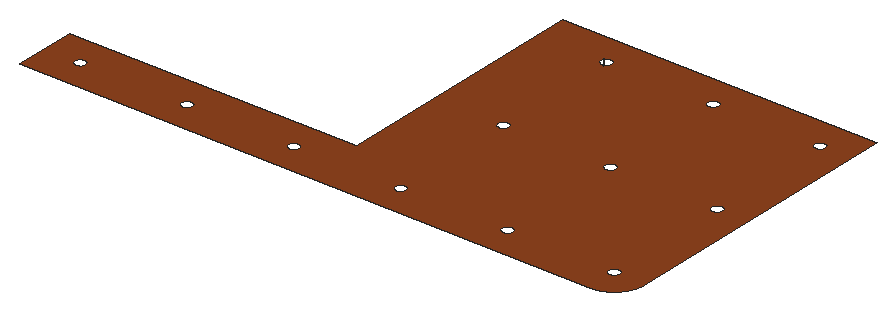
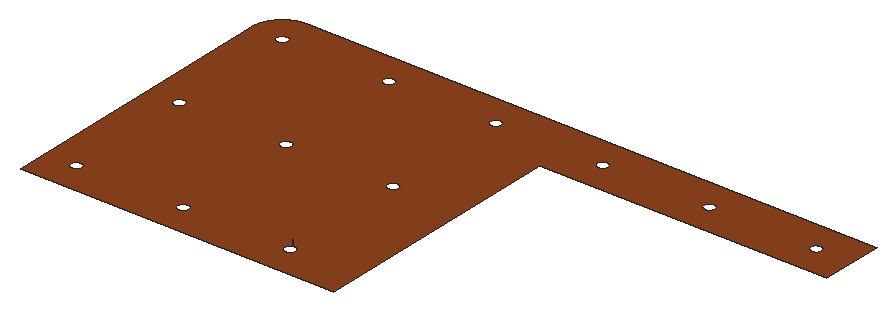
# SketchUp Ruby script. Lengths in inches.
U = 1.inch
M = Sketchup.active_model
def pt(a) = Geom::Point3d.new(a.map { |v| v * U })
def face(e, loops, mat)
  f = e.add_face(loops[0].map { |a| pt(a) })
  loops[1..].each { |l| e.add_face(l.map { |a| pt(a) }).erase! }
  f.material = f.back_material = mat if mat
  f
end
# faces: each face lists its corners as indices into pts; further lists are holes
def faces(e, pts, list, mat = nil) = list.each { |f| face(e, (f[0].is_a?(Array) ? f : [f]).map { |l| l.map { |i| pts[i] } }, mat) }
# xy, xz, yz: faces in a plane at the given z, y or x. An outline is a flat list of corners, or four numbers for a rectangle; further outlines are holes
def ring(l) = l.size == 4 ? [[l[0], l[1]], [l[2], l[1]], [l[2], l[3]], [l[0], l[3]]] : l.each_slice(2).to_a
def flat(e, list, mat, &to3) = list.each { |f| face(e, (f[0].is_a?(Array) ? f : [f]).map { |l| ring(l).map { |u, v| to3.(u, v) } }, mat) }
def xy(e, z, list, mat = nil) = flat(e, list, mat) { |x, y| [x, y, z] }
def xz(e, y, list, mat = nil) = flat(e, list, mat) { |x, z| [x, y, z] }
def yz(e, x, list, mat = nil) = flat(e, list, mat) { |y, z| [x, y, z] }
def lines(e, pts, list) = list.each { |a, b| e.add_line(pt(pts[a]), pt(pts[b])) }
# prism: a flat outline (further loops are holes) pulled along v
def prism(e, loops, v, mat = nil)
  f = face(e, loops, mat); d = Geom::Vector3d.new(v.map { |x| x * U })
  f.pushpull(f.normal.samedirection?(d) ? d.length : -d.length)
end
def box(e, o, s, mat = nil) = prism(e, [[o, [o[0] + s[0], o[1], o[2]], [o[0] + s[0], o[1] + s[1], o[2]], [o[0], o[1] + s[1], o[2]]]], [0, 0, s[2]], mat)
def at(x, y, z, deg = 0) = Geom::Transformation.translation(pt([x, y, z])) * Geom::Transformation.rotation(ORIGIN, Z_AXIS, deg.degrees)
def axes(o, x, y, z) = Geom::Transformation.new([*x, 0, *y, 0, *z, 0, *pt(o).to_a, 1])
def part(name) = M.definitions.add(name)
# library, detail: a bought-in or finely detailed component or shape, given as its bounding box
def library(name, o, s) = part(name).tap { |d| box(d.entities, o, s) }
def detail(e, o, s) = box(e.add_group.entities, o, s)
def put(e, d, t, mat = nil) = e.add_instance(d, t).tap { |i| i.material = mat if mat }
def group(e, t, mat = nil) = e.add_group.tap { |g| g.transformation = t; g.material = mat if mat }.entities
root = M.entities
M.materials.add("[Wood Fence]").color = [142, 67, 30]
xy(root,231,[[[32,172,32,204,179,204,179,336,340,336,340,187.79,339.99,187.58,339.99,187.37,339.97,186.95,339.95,186.74,339.93,186.54,339.89,186.12,339.83,185.7,339.8,185.5,339.77,185.29,339.73,185.08,339.69,184.88,339.65,184.67,339.61,184.47,339.56,184.26,339.51,184.0625,339.45,183.86,339.4,183.66,339.22,183.06,339.01,182.46,338.9375,182.27,338.86,182.07,338.78,181.88,338.7,181.68,338.62,181.49,338.35,180.92,338.26,180.74,338.16,180.55,338.0625,180.37,337.96,180.18,337.86,180,337.53,179.46,337.42,179.29,337.3,179.11,337.1875,178.9375,337.07,178.77,336.94,178.6,336.82,178.43,336.69,178.26,336.57,178.09,336.43,177.93,336.17,177.61,335.89,177.29,335.61,176.99,335.46,176.84,335.3125,176.6875,335.16,176.54,335.01,176.39,334.71,176.11,334.39,175.83,334.07,175.57,333.91,175.43,333.74,175.31,333.57,175.18,333.4,175.06,333.23,174.93,333.0625,174.8125,332.89,174.7,332.71,174.58,332.54,174.47,332,174.14,331.82,174.04,331.63,173.9375,331.45,173.84,331.26,173.74,331.08,173.65,330.51,173.38,330.32,173.3,330.12,173.22,329.93,173.14,329.73,173.0625,329.54,172.99,328.94,172.78,328.34,172.6,328.14,172.55,327.9375,172.49,327.74,172.44,327.53,172.39,327.33,172.35,327.12,172.31,326.92,172.27,326.71,172.23,326.5,172.2,326.3,172.17,325.88,172.11,325.46,172.07,325.26,172.05,325.05,172.03,324.63,172.01,324.42,172.01,324.21,172],[214.28,251,214.51,251,214.59,251.01,214.67,251.01,214.75,251.02,214.82,251.03,214.9,251.04,214.98,251.06,215.06,251.07,215.13,251.09,215.21,251.11,215.28,251.13,215.36,251.16,215.43,251.18,215.51,251.21,215.65,251.27,215.72,251.31,215.79,251.34,216,251.46,216.0625,251.5,216.125,251.55,216.19,251.59,216.25,251.64,216.375,251.74,216.43,251.79,216.6,251.96,216.85,252.26,216.89,252.33,216.93,252.39,216.98,252.46,217.01,252.53,217.09,252.67,217.18,252.88,217.21,252.96,217.24,253.03,217.26,253.1,217.29,253.18,217.31,253.26,217.32,253.33,217.36,253.49,217.37,253.5625,217.38,253.64,217.39,253.72,217.39,253.8,217.4,253.875,217.4,254.11,217.39,254.19,217.39,254.27,217.38,254.35,217.37,254.42,217.36,254.5,217.34,254.58,217.33,254.66,217.31,254.73,217.29,254.81,217.27,254.88,217.24,254.96,217.22,255.03,217.1875,255.11,217.16,255.18,217.09,255.32,217.06,255.39,216.94,255.6,216.9,255.66,216.85,255.73,216.81,255.79,216.61,256.03,216.44,256.2,216.14,256.45,216.07,256.49,216.01,256.53,215.9375,256.58,215.87,256.61,215.8,256.65,215.73,256.6875,215.66,256.72,215.52,256.78,215.44,256.8125,215.37,256.84,215.3,256.86,215.22,256.89,215.14,256.91,215.07,256.92,214.91,256.96,214.84,256.97,214.68,256.99,214.6,256.99,214.52,257,214.29,257,214.21,256.99,214.13,256.99,214.05,256.98,213.98,256.97,213.9,256.96,213.82,256.94,213.74,256.93,213.67,256.91,213.59,256.89,213.52,256.87,213.44,256.84,213.37,256.82,213.29,256.79,213.15,256.73,213.08,256.69,213.01,256.66,212.9375,256.62,212.87,256.58,212.8,256.54,212.74,256.5,212.67,256.45,212.61,256.41,212.37,256.21,212.3125,256.15,212.26,256.1,212.2,256.04,211.95,255.74,211.91,255.67,211.87,255.61,211.82,255.54,211.79,255.47,211.71,255.33,211.62,255.12,211.59,255.04,211.5625,254.97,211.54,254.9,211.51,254.82,211.49,254.74,211.48,254.67,211.44,254.51,211.43,254.4375,211.42,254.36,211.41,254.28,211.41,254.2,211.4,254.125,211.4,253.89,211.41,253.81,211.41,253.73,211.42,253.65,211.43,253.58,211.44,253.5,211.46,253.42,211.47,253.34,211.49,253.27,211.51,253.19,211.53,253.12,211.56,253.04,211.58,252.97,211.61,252.89,211.67,252.75,211.71,252.68,211.74,252.61,211.86,252.4,211.9,252.34,211.95,252.27,211.99,252.21,212.19,251.97,212.36,251.8,212.66,251.55,212.73,251.51,212.79,251.47,212.86,251.42,212.93,251.39,213,251.35,213.07,251.3125,213.14,251.28,213.28,251.22,213.36,251.1875,213.43,251.16,213.5,251.14,213.58,251.11,213.66,251.09,213.73,251.08,213.89,251.04,213.96,251.03,214.12,251.01,214.2,251.01],[214.28,317,214.51,317,214.59,317.01,214.67,317.01,214.75,317.02,214.82,317.03,214.9,317.04,214.98,317.06,215.06,317.07,215.13,317.09,215.21,317.11,215.28,317.13,215.36,317.16,215.43,317.18,215.51,317.21,215.65,317.27,215.72,317.31,215.79,317.34,216,317.46,216.0625,317.5,216.125,317.55,216.19,317.59,216.25,317.64,216.375,317.74,216.43,317.79,216.6,317.96,216.85,318.26,216.89,318.33,216.93,318.39,216.98,318.46,217.01,318.53,217.09,318.67,217.18,318.88,217.21,318.96,217.24,319.03,217.26,319.1,217.29,319.18,217.31,319.26,217.32,319.33,217.36,319.49,217.37,319.5625,217.38,319.64,217.39,319.72,217.39,319.8,217.4,319.875,217.4,320.11,217.39,320.19,217.39,320.27,217.38,320.35,217.37,320.42,217.36,320.5,217.34,320.58,217.33,320.66,217.31,320.73,217.29,320.81,217.27,320.88,217.24,320.96,217.22,321.03,217.1875,321.11,217.16,321.18,217.09,321.32,217.06,321.39,216.94,321.6,216.9,321.66,216.85,321.73,216.81,321.79,216.61,322.03,216.44,322.2,216.14,322.45,216.07,322.49,216.01,322.53,215.9375,322.58,215.87,322.61,215.8,322.65,215.73,322.6875,215.66,322.72,215.52,322.78,215.44,322.8125,215.37,322.84,215.3,322.86,215.22,322.89,215.14,322.91,215.07,322.92,214.91,322.96,214.84,322.97,214.68,322.99,214.6,322.99,214.52,323,214.29,323,214.21,322.99,214.13,322.99,214.05,322.98,213.98,322.97,213.9,322.96,213.82,322.94,213.74,322.93,213.67,322.91,213.59,322.89,213.52,322.87,213.44,322.84,213.37,322.82,213.29,322.79,213.15,322.73,213.08,322.69,213.01,322.66,212.9375,322.62,212.87,322.58,212.8,322.54,212.74,322.5,212.67,322.45,212.61,322.41,212.37,322.21,212.3125,322.15,212.26,322.1,212.2,322.04,211.95,321.74,211.91,321.67,211.87,321.61,211.82,321.54,211.79,321.47,211.71,321.33,211.62,321.12,211.59,321.04,211.5625,320.97,211.54,320.9,211.51,320.82,211.49,320.74,211.48,320.67,211.44,320.51,211.43,320.4375,211.42,320.36,211.41,320.28,211.41,320.2,211.4,320.125,211.4,319.89,211.41,319.81,211.41,319.73,211.42,319.65,211.43,319.58,211.44,319.5,211.46,319.42,211.47,319.34,211.49,319.27,211.51,319.19,211.53,319.12,211.56,319.04,211.58,318.97,211.61,318.89,211.67,318.75,211.71,318.68,211.74,318.61,211.86,318.4,211.9,318.34,211.95,318.27,211.99,318.21,212.19,317.97,212.36,317.8,212.66,317.55,212.73,317.51,212.79,317.47,212.86,317.42,212.93,317.39,213,317.35,213.07,317.3125,213.14,317.28,213.28,317.22,213.36,317.1875,213.43,317.16,213.5,317.14,213.58,317.11,213.66,317.09,213.73,317.08,213.89,317.04,213.96,317.03,214.12,317.01,214.2,317.01],[269.08,317,269.3125,317,269.39,317.01,269.47,317.01,269.55,317.02,269.7,317.04,269.78,317.06,269.86,317.07,269.93,317.09,270.01,317.11,270.08,317.13,270.16,317.16,270.23,317.18,270.31,317.21,270.45,317.27,270.52,317.31,270.59,317.34,270.8,317.46,270.86,317.5,270.93,317.55,270.99,317.59,271.23,317.79,271.4,317.96,271.65,318.26,271.69,318.33,271.73,318.39,271.78,318.46,271.81,318.53,271.89,318.67,271.98,318.88,272.01,318.96,272.04,319.03,272.0625,319.1,272.09,319.18,272.11,319.26,272.125,319.33,272.14,319.41,272.16,319.49,272.17,319.5625,272.18,319.64,272.1875,319.72,272.19,319.8,272.2,319.875,272.2,320.11,272.19,320.19,272.1875,320.27,272.18,320.35,272.17,320.42,272.16,320.5,272.14,320.58,272.13,320.66,272.11,320.73,272.09,320.81,272.07,320.88,272.04,320.96,272.02,321.03,271.99,321.11,271.93,321.25,271.89,321.32,271.86,321.39,271.74,321.6,271.7,321.66,271.65,321.73,271.61,321.79,271.41,322.03,271.24,322.2,271.12,322.3,271.0625,322.35,270.9375,322.45,270.87,322.49,270.81,322.53,270.74,322.58,270.67,322.61,270.6,322.65,270.53,322.6875,270.46,322.72,270.32,322.78,270.24,322.8125,270.17,322.84,270.1,322.86,270.02,322.89,269.94,322.91,269.87,322.92,269.71,322.96,269.64,322.97,269.48,322.99,269.4,322.99,269.32,323,269.09,323,269.01,322.99,268.93,322.99,268.85,322.98,268.78,322.97,268.7,322.96,268.62,322.94,268.54,322.93,268.47,322.91,268.39,322.89,268.32,322.87,268.24,322.84,268.17,322.82,268.09,322.79,267.95,322.73,267.88,322.69,267.81,322.66,267.6,322.54,267.54,322.5,267.47,322.45,267.41,322.41,267.17,322.21,267,322.04,266.75,321.74,266.71,321.67,266.67,321.61,266.625,321.54,266.59,321.47,266.51,321.33,266.42,321.12,266.39,321.04,266.36,320.97,266.34,320.9,266.3125,320.82,266.29,320.74,266.28,320.67,266.24,320.51,266.23,320.4375,266.22,320.36,266.21,320.28,266.21,320.2,266.2,320.125,266.2,319.89,266.21,319.81,266.21,319.73,266.22,319.65,266.23,319.58,266.24,319.5,266.26,319.42,266.27,319.34,266.29,319.27,266.3125,319.19,266.33,319.12,266.36,319.04,266.38,318.97,266.41,318.89,266.47,318.75,266.51,318.68,266.54,318.61,266.66,318.4,266.7,318.34,266.75,318.27,266.79,318.21,266.99,317.97,267.16,317.8,267.46,317.55,267.53,317.51,267.59,317.47,267.66,317.42,267.73,317.39,267.8,317.35,267.87,317.3125,267.9375,317.28,268.01,317.25,268.08,317.22,268.16,317.1875,268.23,317.16,268.3,317.14,268.38,317.11,268.46,317.09,268.53,317.08,268.61,317.06,268.6875,317.04,268.76,317.03,268.92,317.01,269,317.01],[323.875,317,324.11,317,324.19,317.01,324.27,317.01,324.35,317.02,324.42,317.03,324.5,317.04,324.58,317.06,324.66,317.07,324.73,317.09,324.81,317.11,324.88,317.13,324.96,317.16,325.03,317.18,325.11,317.21,325.25,317.27,325.32,317.31,325.39,317.34,325.6,317.46,325.66,317.5,325.73,317.55,325.79,317.59,326.03,317.79,326.2,317.96,326.45,318.26,326.49,318.33,326.53,318.39,326.58,318.46,326.61,318.53,326.65,318.6,326.6875,318.67,326.72,318.74,326.78,318.88,326.8125,318.96,326.84,319.03,326.86,319.1,326.89,319.18,326.91,319.26,326.92,319.33,326.96,319.49,326.97,319.5625,326.98,319.64,326.99,319.72,326.99,319.8,327,319.875,327,320.11,326.99,320.19,326.99,320.27,326.98,320.35,326.97,320.42,326.96,320.5,326.94,320.58,326.93,320.66,326.91,320.73,326.89,320.81,326.87,320.88,326.84,320.96,326.82,321.03,326.79,321.11,326.73,321.25,326.69,321.32,326.66,321.39,326.54,321.6,326.5,321.66,326.45,321.73,326.41,321.79,326.21,322.03,326.04,322.2,325.74,322.45,325.67,322.49,325.61,322.53,325.54,322.58,325.47,322.61,325.4,322.65,325.33,322.6875,325.26,322.72,325.12,322.78,325.04,322.8125,324.97,322.84,324.9,322.86,324.82,322.89,324.74,322.91,324.67,322.92,324.51,322.96,324.4375,322.97,324.36,322.98,324.28,322.99,324.2,322.99,324.125,323,323.89,323,323.81,322.99,323.73,322.99,323.65,322.98,323.58,322.97,323.5,322.96,323.42,322.94,323.34,322.93,323.27,322.91,323.19,322.89,323.12,322.87,323.04,322.84,322.97,322.82,322.89,322.79,322.75,322.73,322.68,322.69,322.61,322.66,322.4,322.54,322.34,322.5,322.27,322.45,322.21,322.41,321.97,322.21,321.8,322.04,321.55,321.74,321.51,321.67,321.47,321.61,321.42,321.54,321.39,321.47,321.35,321.4,321.3125,321.33,321.28,321.26,321.22,321.12,321.1875,321.04,321.16,320.97,321.14,320.9,321.11,320.82,321.09,320.74,321.08,320.67,321.04,320.51,321.03,320.4375,321.02,320.36,321.01,320.28,321.01,320.2,321,320.125,321,319.89,321.01,319.81,321.01,319.73,321.02,319.65,321.03,319.58,321.04,319.5,321.06,319.42,321.07,319.34,321.09,319.27,321.11,319.19,321.13,319.12,321.16,319.04,321.18,318.97,321.21,318.89,321.27,318.75,321.31,318.68,321.34,318.61,321.46,318.4,321.5,318.34,321.55,318.27,321.59,318.21,321.79,317.97,321.96,317.8,322.26,317.55,322.33,317.51,322.39,317.47,322.46,317.42,322.53,317.39,322.6,317.35,322.67,317.3125,322.74,317.28,322.88,317.22,322.96,317.1875,323.03,317.16,323.1,317.14,323.18,317.11,323.26,317.09,323.33,317.08,323.49,317.04,323.5625,317.03,323.64,317.02,323.72,317.01,323.8,317.01],[49.875,185,50.11,185,50.19,185.01,50.27,185.01,50.35,185.02,50.42,185.03,50.5,185.04,50.58,185.06,50.66,185.07,50.73,185.09,50.81,185.11,50.88,185.13,50.96,185.16,51.03,185.18,51.11,185.21,51.25,185.27,51.32,185.31,51.39,185.34,51.6,185.46,51.66,185.5,51.73,185.55,51.79,185.59,52.03,185.79,52.2,185.96,52.45,186.26,52.49,186.33,52.53,186.39,52.58,186.46,52.61,186.53,52.65,186.6,52.6875,186.67,52.72,186.74,52.78,186.88,52.8125,186.96,52.84,187.03,52.86,187.1,52.89,187.18,52.91,187.26,52.92,187.33,52.96,187.49,52.97,187.5625,52.98,187.64,52.99,187.72,52.99,187.8,53,187.875,53,188.11,52.99,188.19,52.99,188.27,52.98,188.35,52.97,188.42,52.96,188.5,52.94,188.58,52.93,188.66,52.91,188.73,52.89,188.81,52.87,188.88,52.84,188.96,52.82,189.03,52.79,189.11,52.73,189.25,52.69,189.32,52.66,189.39,52.54,189.6,52.5,189.66,52.45,189.73,52.41,189.79,52.21,190.03,52.04,190.2,51.74,190.45,51.67,190.49,51.61,190.53,51.54,190.58,51.47,190.61,51.4,190.65,51.33,190.6875,51.26,190.72,51.12,190.78,51.04,190.8125,50.97,190.84,50.9,190.86,50.82,190.89,50.74,190.91,50.67,190.92,50.51,190.96,50.4375,190.97,50.36,190.98,50.28,190.99,50.2,190.99,50.125,191,49.89,191,49.81,190.99,49.73,190.99,49.65,190.98,49.58,190.97,49.5,190.96,49.42,190.94,49.34,190.93,49.27,190.91,49.19,190.89,49.12,190.87,49.04,190.84,48.97,190.82,48.89,190.79,48.75,190.73,48.68,190.69,48.61,190.66,48.4,190.54,48.34,190.5,48.27,190.45,48.21,190.41,47.97,190.21,47.8,190.04,47.55,189.74,47.51,189.67,47.47,189.61,47.42,189.54,47.39,189.47,47.35,189.4,47.3125,189.33,47.28,189.26,47.22,189.12,47.1875,189.04,47.16,188.97,47.14,188.9,47.11,188.82,47.09,188.74,47.08,188.67,47.04,188.51,47.03,188.4375,47.02,188.36,47.01,188.28,47.01,188.2,47,188.125,47,187.89,47.01,187.81,47.01,187.73,47.02,187.65,47.03,187.58,47.04,187.5,47.06,187.42,47.07,187.34,47.09,187.27,47.11,187.19,47.13,187.12,47.16,187.04,47.18,186.97,47.21,186.89,47.27,186.75,47.31,186.68,47.34,186.61,47.46,186.4,47.5,186.34,47.55,186.27,47.59,186.21,47.79,185.97,47.96,185.8,48.26,185.55,48.33,185.51,48.39,185.47,48.46,185.42,48.53,185.39,48.6,185.35,48.67,185.3125,48.74,185.28,48.88,185.22,48.96,185.1875,49.03,185.16,49.1,185.14,49.18,185.11,49.26,185.09,49.33,185.08,49.49,185.04,49.5625,185.03,49.64,185.02,49.72,185.01,49.8,185.01],[269.08,251,269.3125,251,269.39,251.01,269.47,251.01,269.55,251.02,269.7,251.04,269.78,251.06,269.86,251.07,269.93,251.09,270.01,251.11,270.08,251.13,270.16,251.16,270.23,251.18,270.31,251.21,270.45,251.27,270.52,251.31,270.59,251.34,270.8,251.46,270.86,251.5,270.93,251.55,270.99,251.59,271.23,251.79,271.4,251.96,271.65,252.26,271.69,252.33,271.73,252.39,271.78,252.46,271.81,252.53,271.89,252.67,271.98,252.88,272.01,252.96,272.04,253.03,272.0625,253.1,272.09,253.18,272.11,253.26,272.125,253.33,272.14,253.41,272.16,253.49,272.17,253.5625,272.18,253.64,272.1875,253.72,272.19,253.8,272.2,253.875,272.2,254.11,272.19,254.19,272.1875,254.27,272.18,254.35,272.17,254.42,272.16,254.5,272.14,254.58,272.13,254.66,272.11,254.73,272.09,254.81,272.07,254.88,272.04,254.96,272.02,255.03,271.99,255.11,271.93,255.25,271.89,255.32,271.86,255.39,271.74,255.6,271.7,255.66,271.65,255.73,271.61,255.79,271.41,256.03,271.24,256.2,271.12,256.3,271.0625,256.35,270.9375,256.45,270.87,256.49,270.81,256.53,270.74,256.58,270.67,256.61,270.6,256.65,270.53,256.6875,270.46,256.72,270.32,256.78,270.24,256.8125,270.17,256.84,270.1,256.86,270.02,256.89,269.94,256.91,269.87,256.92,269.71,256.96,269.64,256.97,269.48,256.99,269.4,256.99,269.32,257,269.09,257,269.01,256.99,268.93,256.99,268.85,256.98,268.78,256.97,268.7,256.96,268.62,256.94,268.54,256.93,268.47,256.91,268.39,256.89,268.32,256.87,268.24,256.84,268.17,256.82,268.09,256.79,267.95,256.73,267.88,256.69,267.81,256.66,267.6,256.54,267.54,256.5,267.47,256.45,267.41,256.41,267.17,256.21,267,256.04,266.75,255.74,266.71,255.67,266.67,255.61,266.625,255.54,266.59,255.47,266.51,255.33,266.42,255.12,266.39,255.04,266.36,254.97,266.34,254.9,266.3125,254.82,266.29,254.74,266.28,254.67,266.24,254.51,266.23,254.4375,266.22,254.36,266.21,254.28,266.21,254.2,266.2,254.125,266.2,253.89,266.21,253.81,266.21,253.73,266.22,253.65,266.23,253.58,266.24,253.5,266.26,253.42,266.27,253.34,266.29,253.27,266.3125,253.19,266.33,253.12,266.36,253.04,266.38,252.97,266.41,252.89,266.47,252.75,266.51,252.68,266.54,252.61,266.66,252.4,266.7,252.34,266.75,252.27,266.79,252.21,266.99,251.97,267.16,251.8,267.46,251.55,267.53,251.51,267.59,251.47,267.66,251.42,267.73,251.39,267.8,251.35,267.87,251.3125,267.9375,251.28,268.01,251.25,268.08,251.22,268.16,251.1875,268.23,251.16,268.3,251.14,268.38,251.11,268.46,251.09,268.53,251.08,268.61,251.06,268.6875,251.04,268.76,251.03,268.92,251.01,269,251.01],[323.875,251,324.11,251,324.19,251.01,324.27,251.01,324.35,251.02,324.42,251.03,324.5,251.04,324.58,251.06,324.66,251.07,324.73,251.09,324.81,251.11,324.88,251.13,324.96,251.16,325.03,251.18,325.11,251.21,325.25,251.27,325.32,251.31,325.39,251.34,325.6,251.46,325.66,251.5,325.73,251.55,325.79,251.59,326.03,251.79,326.2,251.96,326.45,252.26,326.49,252.33,326.53,252.39,326.58,252.46,326.61,252.53,326.65,252.6,326.6875,252.67,326.72,252.74,326.78,252.88,326.8125,252.96,326.84,253.03,326.86,253.1,326.89,253.18,326.91,253.26,326.92,253.33,326.96,253.49,326.97,253.5625,326.98,253.64,326.99,253.72,326.99,253.8,327,253.875,327,254.11,326.99,254.19,326.99,254.27,326.98,254.35,326.97,254.42,326.96,254.5,326.94,254.58,326.93,254.66,326.91,254.73,326.89,254.81,326.87,254.88,326.84,254.96,326.82,255.03,326.79,255.11,326.73,255.25,326.69,255.32,326.66,255.39,326.54,255.6,326.5,255.66,326.45,255.73,326.41,255.79,326.21,256.03,326.04,256.2,325.74,256.45,325.67,256.49,325.61,256.53,325.54,256.58,325.47,256.61,325.4,256.65,325.33,256.6875,325.26,256.72,325.12,256.78,325.04,256.8125,324.97,256.84,324.9,256.86,324.82,256.89,324.74,256.91,324.67,256.92,324.51,256.96,324.4375,256.97,324.36,256.98,324.28,256.99,324.2,256.99,324.125,257,323.89,257,323.81,256.99,323.73,256.99,323.65,256.98,323.58,256.97,323.5,256.96,323.42,256.94,323.34,256.93,323.27,256.91,323.19,256.89,323.12,256.87,323.04,256.84,322.97,256.82,322.89,256.79,322.75,256.73,322.68,256.69,322.61,256.66,322.4,256.54,322.34,256.5,322.27,256.45,322.21,256.41,321.97,256.21,321.8,256.04,321.55,255.74,321.51,255.67,321.47,255.61,321.42,255.54,321.39,255.47,321.35,255.4,321.3125,255.33,321.28,255.26,321.22,255.12,321.1875,255.04,321.16,254.97,321.14,254.9,321.11,254.82,321.09,254.74,321.08,254.67,321.04,254.51,321.03,254.4375,321.02,254.36,321.01,254.28,321.01,254.2,321,254.125,321,253.89,321.01,253.81,321.01,253.73,321.02,253.65,321.03,253.58,321.04,253.5,321.06,253.42,321.07,253.34,321.09,253.27,321.11,253.19,321.13,253.12,321.16,253.04,321.18,252.97,321.21,252.89,321.27,252.75,321.31,252.68,321.34,252.61,321.46,252.4,321.5,252.34,321.55,252.27,321.59,252.21,321.79,251.97,321.96,251.8,322.26,251.55,322.33,251.51,322.39,251.47,322.46,251.42,322.53,251.39,322.6,251.35,322.67,251.3125,322.74,251.28,322.88,251.22,322.96,251.1875,323.03,251.16,323.1,251.14,323.18,251.11,323.26,251.09,323.33,251.08,323.49,251.04,323.5625,251.03,323.64,251.02,323.72,251.01,323.8,251.01],[269.08,185,269.3125,185,269.39,185.01,269.47,185.01,269.55,185.02,269.7,185.04,269.78,185.06,269.86,185.07,269.93,185.09,270.01,185.11,270.08,185.13,270.16,185.16,270.23,185.18,270.31,185.21,270.45,185.27,270.52,185.31,270.59,185.34,270.8,185.46,270.86,185.5,270.93,185.55,270.99,185.59,271.23,185.79,271.4,185.96,271.65,186.26,271.69,186.33,271.73,186.39,271.78,186.46,271.81,186.53,271.89,186.67,271.98,186.88,272.01,186.96,272.04,187.03,272.0625,187.1,272.09,187.18,272.11,187.26,272.125,187.33,272.14,187.41,272.16,187.49,272.17,187.5625,272.18,187.64,272.1875,187.72,272.19,187.8,272.2,187.875,272.2,188.11,272.19,188.19,272.1875,188.27,272.18,188.35,272.17,188.42,272.16,188.5,272.14,188.58,272.13,188.66,272.11,188.73,272.09,188.81,272.07,188.88,272.04,188.96,272.02,189.03,271.99,189.11,271.93,189.25,271.89,189.32,271.86,189.39,271.74,189.6,271.7,189.66,271.65,189.73,271.61,189.79,271.41,190.03,271.24,190.2,271.12,190.3,271.0625,190.35,270.9375,190.45,270.87,190.49,270.81,190.53,270.74,190.58,270.67,190.61,270.6,190.65,270.53,190.6875,270.46,190.72,270.32,190.78,270.24,190.8125,270.17,190.84,270.1,190.86,270.02,190.89,269.94,190.91,269.87,190.92,269.71,190.96,269.64,190.97,269.48,190.99,269.4,190.99,269.32,191,269.09,191,269.01,190.99,268.93,190.99,268.85,190.98,268.78,190.97,268.7,190.96,268.62,190.94,268.54,190.93,268.47,190.91,268.39,190.89,268.32,190.87,268.24,190.84,268.17,190.82,268.09,190.79,267.95,190.73,267.88,190.69,267.81,190.66,267.6,190.54,267.54,190.5,267.47,190.45,267.41,190.41,267.17,190.21,267,190.04,266.75,189.74,266.71,189.67,266.67,189.61,266.625,189.54,266.59,189.47,266.51,189.33,266.42,189.12,266.39,189.04,266.36,188.97,266.34,188.9,266.3125,188.82,266.29,188.74,266.28,188.67,266.24,188.51,266.23,188.4375,266.22,188.36,266.21,188.28,266.21,188.2,266.2,188.125,266.2,187.89,266.21,187.81,266.21,187.73,266.22,187.65,266.23,187.58,266.24,187.5,266.26,187.42,266.27,187.34,266.29,187.27,266.3125,187.19,266.33,187.12,266.36,187.04,266.38,186.97,266.41,186.89,266.47,186.75,266.51,186.68,266.54,186.61,266.66,186.4,266.7,186.34,266.75,186.27,266.79,186.21,266.99,185.97,267.16,185.8,267.46,185.55,267.53,185.51,267.59,185.47,267.66,185.42,267.73,185.39,267.8,185.35,267.87,185.3125,267.9375,185.28,268.01,185.25,268.08,185.22,268.16,185.1875,268.23,185.16,268.3,185.14,268.38,185.11,268.46,185.09,268.53,185.08,268.61,185.06,268.6875,185.04,268.76,185.03,268.92,185.01,269,185.01],[323.875,185,324.11,185,324.19,185.01,324.27,185.01,324.35,185.02,324.42,185.03,324.5,185.04,324.58,185.06,324.66,185.07,324.73,185.09,324.81,185.11,324.88,185.13,324.96,185.16,325.03,185.18,325.11,185.21,325.25,185.27,325.32,185.31,325.39,185.34,325.6,185.46,325.66,185.5,325.73,185.55,325.79,185.59,326.03,185.79,326.2,185.96,326.45,186.26,326.49,186.33,326.53,186.39,326.58,186.46,326.61,186.53,326.65,186.6,326.6875,186.67,326.72,186.74,326.78,186.88,326.8125,186.96,326.84,187.03,326.86,187.1,326.89,187.18,326.91,187.26,326.92,187.33,326.96,187.49,326.97,187.5625,326.98,187.64,326.99,187.72,326.99,187.8,327,187.875,327,188.11,326.99,188.19,326.99,188.27,326.98,188.35,326.97,188.42,326.96,188.5,326.94,188.58,326.93,188.66,326.91,188.73,326.89,188.81,326.87,188.88,326.84,188.96,326.82,189.03,326.79,189.11,326.73,189.25,326.69,189.32,326.66,189.39,326.54,189.6,326.5,189.66,326.45,189.73,326.41,189.79,326.21,190.03,326.04,190.2,325.74,190.45,325.67,190.49,325.61,190.53,325.54,190.58,325.47,190.61,325.4,190.65,325.33,190.6875,325.26,190.72,325.12,190.78,325.04,190.8125,324.97,190.84,324.9,190.86,324.82,190.89,324.74,190.91,324.67,190.92,324.51,190.96,324.4375,190.97,324.36,190.98,324.28,190.99,324.2,190.99,324.125,191,323.89,191,323.81,190.99,323.73,190.99,323.65,190.98,323.58,190.97,323.5,190.96,323.42,190.94,323.34,190.93,323.27,190.91,323.19,190.89,323.12,190.87,323.04,190.84,322.97,190.82,322.89,190.79,322.75,190.73,322.68,190.69,322.61,190.66,322.4,190.54,322.34,190.5,322.27,190.45,322.21,190.41,321.97,190.21,321.8,190.04,321.55,189.74,321.51,189.67,321.47,189.61,321.42,189.54,321.39,189.47,321.35,189.4,321.3125,189.33,321.28,189.26,321.22,189.12,321.1875,189.04,321.16,188.97,321.14,188.9,321.11,188.82,321.09,188.74,321.08,188.67,321.04,188.51,321.03,188.4375,321.02,188.36,321.01,188.28,321.01,188.2,321,188.125,321,187.89,321.01,187.81,321.01,187.73,321.02,187.65,321.03,187.58,321.04,187.5,321.06,187.42,321.07,187.34,321.09,187.27,321.11,187.19,321.13,187.12,321.16,187.04,321.18,186.97,321.21,186.89,321.27,186.75,321.31,186.68,321.34,186.61,321.46,186.4,321.5,186.34,321.55,186.27,321.59,186.21,321.79,185.97,321.96,185.8,322.26,185.55,322.33,185.51,322.39,185.47,322.46,185.42,322.53,185.39,322.6,185.35,322.67,185.3125,322.74,185.28,322.88,185.22,322.96,185.1875,323.03,185.16,323.1,185.14,323.18,185.11,323.26,185.09,323.33,185.08,323.49,185.04,323.5625,185.03,323.64,185.02,323.72,185.01,323.8,185.01],[104.68,185,104.91,185,104.99,185.01,105.07,185.01,105.15,185.02,105.22,185.03,105.3,185.04,105.38,185.06,105.46,185.07,105.53,185.09,105.61,185.11,105.68,185.13,105.76,185.16,105.83,185.18,105.91,185.21,106.05,185.27,106.12,185.31,106.19,185.34,106.4,185.46,106.46,185.5,106.53,185.55,106.59,185.59,106.83,185.79,107,185.96,107.25,186.26,107.29,186.33,107.33,186.39,107.375,186.46,107.41,186.53,107.49,186.67,107.58,186.88,107.61,186.96,107.64,187.03,107.66,187.1,107.6875,187.18,107.71,187.26,107.72,187.33,107.76,187.49,107.77,187.5625,107.78,187.64,107.79,187.72,107.79,187.8,107.8,187.875,107.8,188.11,107.79,188.19,107.79,188.27,107.78,188.35,107.77,188.42,107.76,188.5,107.74,188.58,107.73,188.66,107.71,188.73,107.6875,188.81,107.67,188.88,107.64,188.96,107.62,189.03,107.59,189.11,107.53,189.25,107.49,189.32,107.46,189.39,107.34,189.6,107.3,189.66,107.25,189.73,107.21,189.79,107.01,190.03,106.84,190.2,106.54,190.45,106.47,190.49,106.41,190.53,106.34,190.58,106.27,190.61,106.2,190.65,106.13,190.6875,106.0625,190.72,105.99,190.75,105.92,190.78,105.84,190.8125,105.77,190.84,105.7,190.86,105.62,190.89,105.54,190.91,105.47,190.92,105.39,190.94,105.3125,190.96,105.24,190.97,105.08,190.99,105,190.99,104.92,191,104.6875,191,104.61,190.99,104.53,190.99,104.45,190.98,104.3,190.96,104.22,190.94,104.14,190.93,104.07,190.91,103.99,190.89,103.92,190.87,103.84,190.84,103.77,190.82,103.69,190.79,103.55,190.73,103.48,190.69,103.41,190.66,103.2,190.54,103.14,190.5,103.07,190.45,103.01,190.41,102.77,190.21,102.6,190.04,102.35,189.74,102.31,189.67,102.27,189.61,102.22,189.54,102.19,189.47,102.11,189.33,102.02,189.12,101.99,189.04,101.96,188.97,101.9375,188.9,101.91,188.82,101.89,188.74,101.875,188.67,101.86,188.59,101.84,188.51,101.83,188.4375,101.82,188.36,101.8125,188.28,101.81,188.2,101.8,188.125,101.8,187.89,101.81,187.81,101.8125,187.73,101.82,187.65,101.83,187.58,101.84,187.5,101.86,187.42,101.87,187.34,101.89,187.27,101.91,187.19,101.93,187.12,101.96,187.04,101.98,186.97,102.01,186.89,102.07,186.75,102.11,186.68,102.14,186.61,102.26,186.4,102.3,186.34,102.35,186.27,102.39,186.21,102.59,185.97,102.76,185.8,102.88,185.7,102.9375,185.65,103.0625,185.55,103.13,185.51,103.19,185.47,103.26,185.42,103.33,185.39,103.4,185.35,103.47,185.3125,103.54,185.28,103.68,185.22,103.76,185.1875,103.83,185.16,103.9,185.14,103.98,185.11,104.06,185.09,104.13,185.08,104.29,185.04,104.36,185.03,104.52,185.01,104.6,185.01],[159.48,185,159.71,185,159.79,185.01,159.87,185.01,159.95,185.02,160.02,185.03,160.1,185.04,160.18,185.06,160.26,185.07,160.33,185.09,160.41,185.11,160.48,185.13,160.56,185.16,160.63,185.18,160.71,185.21,160.85,185.27,160.92,185.31,160.99,185.34,161.0625,185.38,161.13,185.42,161.2,185.46,161.26,185.5,161.33,185.55,161.39,185.59,161.63,185.79,161.6875,185.85,161.74,185.9,161.8,185.96,162.05,186.26,162.09,186.33,162.13,186.39,162.18,186.46,162.21,186.53,162.29,186.67,162.38,186.88,162.41,186.96,162.4375,187.03,162.46,187.1,162.49,187.18,162.51,187.26,162.52,187.33,162.56,187.49,162.57,187.5625,162.58,187.64,162.59,187.72,162.59,187.8,162.6,187.875,162.6,188.11,162.59,188.19,162.59,188.27,162.58,188.35,162.57,188.42,162.56,188.5,162.54,188.58,162.53,188.66,162.51,188.73,162.49,188.81,162.47,188.88,162.44,188.96,162.42,189.03,162.39,189.11,162.33,189.25,162.29,189.32,162.26,189.39,162.14,189.6,162.1,189.66,162.05,189.73,162.01,189.79,161.81,190.03,161.64,190.2,161.34,190.45,161.27,190.49,161.21,190.53,161.14,190.58,161.07,190.61,161,190.65,160.93,190.6875,160.86,190.72,160.72,190.78,160.64,190.8125,160.57,190.84,160.5,190.86,160.42,190.89,160.34,190.91,160.27,190.92,160.11,190.96,160.04,190.97,159.88,190.99,159.8,190.99,159.72,191,159.49,191,159.41,190.99,159.33,190.99,159.25,190.98,159.18,190.97,159.1,190.96,159.02,190.94,158.94,190.93,158.87,190.91,158.79,190.89,158.72,190.87,158.64,190.84,158.57,190.82,158.49,190.79,158.35,190.73,158.28,190.69,158.21,190.66,158,190.54,157.9375,190.5,157.875,190.45,157.81,190.41,157.75,190.36,157.625,190.26,157.57,190.21,157.4,190.04,157.15,189.74,157.11,189.67,157.07,189.61,157.02,189.54,156.99,189.47,156.91,189.33,156.82,189.12,156.79,189.04,156.76,188.97,156.74,188.9,156.71,188.82,156.69,188.74,156.68,188.67,156.64,188.51,156.63,188.4375,156.62,188.36,156.61,188.28,156.61,188.2,156.6,188.125,156.6,187.89,156.61,187.81,156.61,187.73,156.62,187.65,156.63,187.58,156.64,187.5,156.66,187.42,156.67,187.34,156.69,187.27,156.71,187.19,156.73,187.12,156.76,187.04,156.78,186.97,156.8125,186.89,156.84,186.82,156.91,186.68,156.94,186.61,157.06,186.4,157.1,186.34,157.15,186.27,157.19,186.21,157.39,185.97,157.56,185.8,157.86,185.55,157.93,185.51,157.99,185.47,158.0625,185.42,158.13,185.39,158.2,185.35,158.27,185.3125,158.34,185.28,158.48,185.22,158.56,185.1875,158.63,185.16,158.7,185.14,158.78,185.11,158.86,185.09,158.93,185.08,159.09,185.04,159.16,185.03,159.32,185.01,159.4,185.01],[214.28,185,214.51,185,214.59,185.01,214.67,185.01,214.75,185.02,214.82,185.03,214.9,185.04,214.98,185.06,215.06,185.07,215.13,185.09,215.21,185.11,215.28,185.13,215.36,185.16,215.43,185.18,215.51,185.21,215.65,185.27,215.72,185.31,215.79,185.34,216,185.46,216.0625,185.5,216.125,185.55,216.19,185.59,216.25,185.64,216.375,185.74,216.43,185.79,216.6,185.96,216.85,186.26,216.89,186.33,216.93,186.39,216.98,186.46,217.01,186.53,217.09,186.67,217.18,186.88,217.21,186.96,217.24,187.03,217.26,187.1,217.29,187.18,217.31,187.26,217.32,187.33,217.36,187.49,217.37,187.5625,217.38,187.64,217.39,187.72,217.39,187.8,217.4,187.875,217.4,188.11,217.39,188.19,217.39,188.27,217.38,188.35,217.37,188.42,217.36,188.5,217.34,188.58,217.33,188.66,217.31,188.73,217.29,188.81,217.27,188.88,217.24,188.96,217.22,189.03,217.1875,189.11,217.16,189.18,217.09,189.32,217.06,189.39,216.94,189.6,216.9,189.66,216.85,189.73,216.81,189.79,216.61,190.03,216.44,190.2,216.14,190.45,216.07,190.49,216.01,190.53,215.9375,190.58,215.87,190.61,215.8,190.65,215.73,190.6875,215.66,190.72,215.52,190.78,215.44,190.8125,215.37,190.84,215.3,190.86,215.22,190.89,215.14,190.91,215.07,190.92,214.91,190.96,214.84,190.97,214.68,190.99,214.6,190.99,214.52,191,214.29,191,214.21,190.99,214.13,190.99,214.05,190.98,213.98,190.97,213.9,190.96,213.82,190.94,213.74,190.93,213.67,190.91,213.59,190.89,213.52,190.87,213.44,190.84,213.37,190.82,213.29,190.79,213.15,190.73,213.08,190.69,213.01,190.66,212.9375,190.62,212.87,190.58,212.8,190.54,212.74,190.5,212.67,190.45,212.61,190.41,212.37,190.21,212.3125,190.15,212.26,190.1,212.2,190.04,211.95,189.74,211.91,189.67,211.87,189.61,211.82,189.54,211.79,189.47,211.71,189.33,211.62,189.12,211.59,189.04,211.5625,188.97,211.54,188.9,211.51,188.82,211.49,188.74,211.48,188.67,211.44,188.51,211.43,188.4375,211.42,188.36,211.41,188.28,211.41,188.2,211.4,188.125,211.4,187.89,211.41,187.81,211.41,187.73,211.42,187.65,211.43,187.58,211.44,187.5,211.46,187.42,211.47,187.34,211.49,187.27,211.51,187.19,211.53,187.12,211.56,187.04,211.58,186.97,211.61,186.89,211.67,186.75,211.71,186.68,211.74,186.61,211.86,186.4,211.9,186.34,211.95,186.27,211.99,186.21,212.19,185.97,212.36,185.8,212.66,185.55,212.73,185.51,212.79,185.47,212.86,185.42,212.93,185.39,213,185.35,213.07,185.3125,213.14,185.28,213.28,185.22,213.36,185.1875,213.43,185.16,213.5,185.14,213.58,185.11,213.66,185.09,213.73,185.08,213.89,185.04,213.96,185.03,214.12,185.01,214.2,185.01]]],"[Wood Fence]")
p = [[215.21,317.11,231],[215.13,317.09,231],[215.13,317.09,234],[215.21,317.11,234]]
faces(root,p,[[0,1,2,3]])
